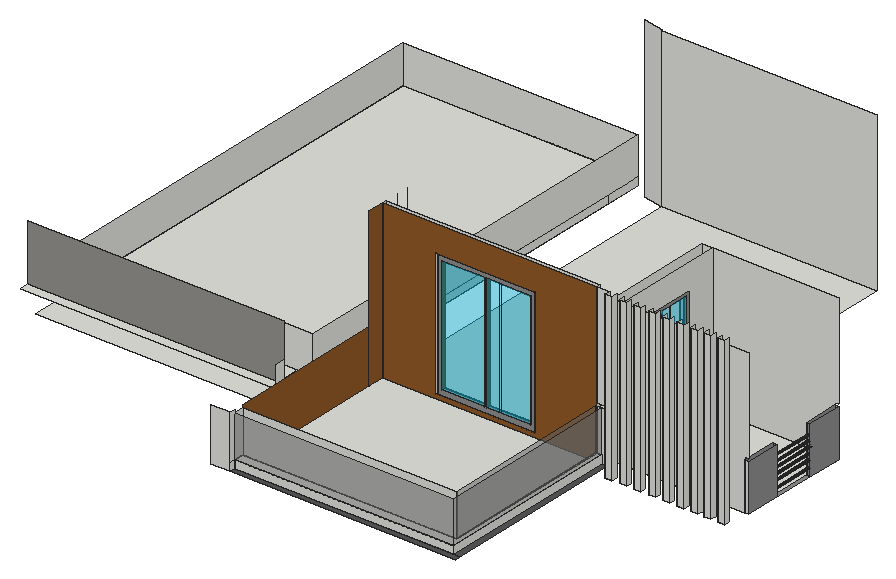
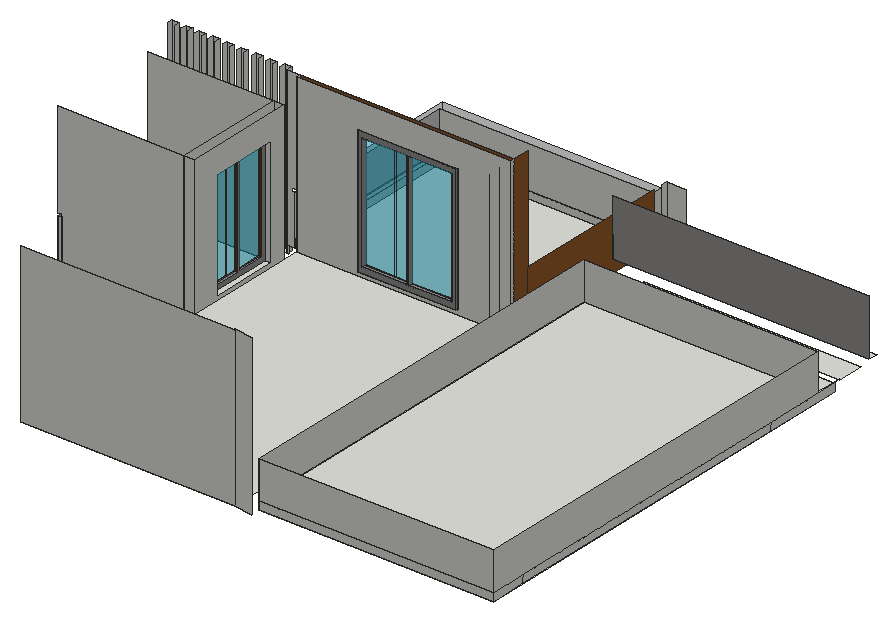
# SketchUp Ruby script. Lengths in inches.
U = 1.inch
M = Sketchup.active_model
def pt(a) = Geom::Point3d.new(a.map { |v| v * U })
def face(e, loops, mat)
  f = e.add_face(loops[0].map { |a| pt(a) })
  loops[1..].each { |l| e.add_face(l.map { |a| pt(a) }).erase! }
  f.material = f.back_material = mat if mat
  f
end
# faces: each face lists its corners as indices into pts; further lists are holes
def faces(e, pts, list, mat = nil) = list.each { |f| face(e, (f[0].is_a?(Array) ? f : [f]).map { |l| l.map { |i| pts[i] } }, mat) }
# xy, xz, yz: faces in a plane at the given z, y or x. An outline is a flat list of corners, or four numbers for a rectangle; further outlines are holes
def ring(l) = l.size == 4 ? [[l[0], l[1]], [l[2], l[1]], [l[2], l[3]], [l[0], l[3]]] : l.each_slice(2).to_a
def flat(e, list, mat, &to3) = list.each { |f| face(e, (f[0].is_a?(Array) ? f : [f]).map { |l| ring(l).map { |u, v| to3.(u, v) } }, mat) }
def xy(e, z, list, mat = nil) = flat(e, list, mat) { |x, y| [x, y, z] }
def xz(e, y, list, mat = nil) = flat(e, list, mat) { |x, z| [x, y, z] }
def yz(e, x, list, mat = nil) = flat(e, list, mat) { |y, z| [x, y, z] }
def lines(e, pts, list) = list.each { |a, b| e.add_line(pt(pts[a]), pt(pts[b])) }
# prism: a flat outline (further loops are holes) pulled along v
def prism(e, loops, v, mat = nil)
  f = face(e, loops, mat); d = Geom::Vector3d.new(v.map { |x| x * U })
  f.pushpull(f.normal.samedirection?(d) ? d.length : -d.length)
end
def box(e, o, s, mat = nil) = prism(e, [[o, [o[0] + s[0], o[1], o[2]], [o[0] + s[0], o[1] + s[1], o[2]], [o[0], o[1] + s[1], o[2]]]], [0, 0, s[2]], mat)
def at(x, y, z, deg = 0) = Geom::Transformation.translation(pt([x, y, z])) * Geom::Transformation.rotation(ORIGIN, Z_AXIS, deg.degrees)
def axes(o, x, y, z) = Geom::Transformation.new([*x, 0, *y, 0, *z, 0, *pt(o).to_a, 1])
def part(name) = M.definitions.add(name)
# library, detail: a bought-in or finely detailed component or shape, given as its bounding box
def library(name, o, s) = part(name).tap { |d| box(d.entities, o, s) }
def detail(e, o, s) = box(e.add_group.entities, o, s)
def put(e, d, t, mat = nil) = e.add_instance(d, t).tap { |i| i.material = mat if mat }
def group(e, t, mat = nil) = e.add_group.tap { |g| g.transformation = t; g.material = mat if mat }.entities
root = M.entities
M.materials.add("[Color C08]2").color = [102, 51, 0]
M.materials.add("[Color M04]").color = [142, 142, 142]
M.materials.add("[Color M06]").color = [86, 86, 86]
M.materials.add("[Color M07]").color = [58, 58, 58]
M.materials.add("[Granite Light Gray]").color = [149, 148, 144]
M.materials.add("[Translucent Glass Gray]").color = [128, 128, 128]
M.materials["[Translucent Glass Gray]"].alpha = 0.5
M.materials.add("[Translucent Glass Tinted]").color = [8, 201, 241]
M.materials["[Translucent Glass Tinted]"].alpha = 0.48
M.materials.add("[Wood Floor Parquet]").color = [145, 89, 39]
c1 = part("Group\#7")
xy(c1.entities,0,[[0,0,91.875,6]],"[Color C08]2")
xy(c1.entities,4.0625,[[4.0625,0,44.34,6],[46.04,0,87.8125,6]],"[Color M04]")
xy(c1.entities,94.75,[[4.0625,0,44.34,6],[46.04,0,87.8125,6]],"[Color M04]")
xy(c1.entities,98.8125,[[0,0,91.875,6]],"[Color M04]")
xz(c1.entities,0,[[[0,0,91.875,98.8125],[46.04,4.0625,87.8125,94.75],[4.0625,4.0625,44.34,94.75]]],"[Color M04]")
xz(c1.entities,0,[[4.0625,4.0625,44.34,94.75],[46.04,4.0625,58.41,94.75],[58.41,4.0625,60.1,94.75],[60.1,4.0625,87.8125,94.75]],"[Translucent Glass Tinted]")
xz(c1.entities,6,[[[0,0,91.875,98.8125],[46.04,4.0625,87.8125,94.75],[4.0625,4.0625,44.34,94.75]]],"[Color M04]")
yz(c1.entities,0,[[0,0,6,98.8125]],"[Color M04]")
yz(c1.entities,4.0625,[[0,4.0625,6,94.75]],"[Color C08]2")
yz(c1.entities,44.34,[[0,4.0625,6,94.75]],"[Color M04]")
yz(c1.entities,46.04,[[0,4.0625,6,94.75]],"[Color C08]2")
yz(c1.entities,87.8125,[[0,4.0625,6,94.75]],"[Color M04]")
yz(c1.entities,91.875,[[0,0,6,98.8125]],"[Color M04]")
xy(root,232.19,[[411.38,417.2,416.8,421.2],[422.38,417.2,427.8,421.2],[433.38,417.2,438.8,421.2],[444.38,417.2,449.8,421.2],[455.38,417.2,460.8,421.2],
  [466.38,417.2,471.8,421.2],[477,417.2,482.43,421.2],[487,417.2,492.43,421.2],[497.19,417.2,502.61,421.2]])
xy(root,232.48,[[503.61,435.35,506.53,462.36],[402.3125,435.41,410.3125,521],[410.3125,435.41,503.61,521],[503.61,494.13,506.53,521]])
xy(root,232.48,[[503.61,462.36,506.53,494.13]],"[Color M04]")
xy(root,234.27,[[51.29,358.3125,188.16,364.3125]])
xy(root,237.8125,[[238,280.08,238,287.59,401.5625,287.59,401.5625,421.2,405.5625,421.2,405.5625,280.08],[238,287.59,401.5625,421.2],[238,421.2,401.5625,424.01],[238,424.01,401.5625,688.37]])
xy(root,237.8125,[[238,275.76,410.3125,280.08],[405.5625,280.08,410.3125,421.2]],"[Color M06]")
xy(root,240.32,[[402.3125,448.18,410.3125,499.8]])
xy(root,241.2,[[279.03,421.2,354.66,424.01]])
xy(root,243.375,[[38.1875,364.3125,217,690.87]])
xy(root,243.8125,[[238,280.08,238,287.59,401.5625,287.59,401.5625,421.2,405.5625,421.2,405.5625,280.08],[401.36,287.59,401.5625,421.2]])
xy(root,248.4375,[[39.5625,338.43,205.18,358.3125]])
xy(root,249.375,[[38.1875,364.3125,39.5625,380.8125],[39.5625,364.3125,205.18,380.8125],[205.18,364.3125,217,380.8125],[38.1875,380.8125,217,690.87]])
xy(root,261.375,[[27.5625,338.43,223,345.62]])
xz(root,275.76,[[223,237.8125,238,278.0625]])
xz(root,280.08,[[238,237.8125,405.5625,243.8125]])
xz(root,280.08,[[238,243.8125,405.5625,276.0625]],"[Translucent Glass Gray]")
xz(root,287.59,[[238,237.8125,401.5625,243.8125],[238,243.8125,401.36,276.0625]])
xz(root,345.62,[[27.5625,261.375,223,304.375]],"[Granite Light Gray]")
xz(root,364.3125,[[38.1875,243.375,39.5625,249.375],[39.5625,243.375,205.18,249.375],[205.18,243.375,217,249.375]])
xz(root,380.8125,[[38.1875,249.375,39.5625,278.375],[39.5625,249.375,217,278.375]])
xz(root,417.2,[[411.38,232.19,416.8,357.8125],[422.38,232.19,427.8,357.8125],[433.38,232.19,438.8,357.8125],[444.38,232.19,449.8,357.8125],[455.38,232.19,460.8,357.8125],
  [466.38,232.19,471.8,357.8125],[477,232.19,482.43,357.8125],[487,232.19,492.43,357.8125],[497.19,232.19,502.61,357.8125]])
xz(root,421.2,[[410.3125,232.19,411.38,237.8125],[401.5625,237.8125,405.5625,243.8125],[405.5625,237.8125,411.38,237.8125,411.38,357.8125,401.5625,357.8125,401.5625,278.0625,407.6875,278.0625,407.6875,276.0625,405.5625,276.0625],[401.36,243.8125,401.5625,276.0625],[401.5625,243.8125,405.5625,276.0625]])
xz(root,421.2,[[[238,237.8125,401.5625,237.8125,401.5625,243.8125,401.36,243.8125,401.36,278.0625,401.5625,278.0625,401.5625,357.8125,238,357.8125],[279.03,241.2,354.66,337.83]]],"[Wood Floor Parquet]")
xz(root,424.01,[[[238,237.8125,401.5625,357.8125],[279.03,241.2,354.66,337.83]]])
xz(root,435.35,[[503.61,232.48,506.53,268.48]])
xz(root,435.41,[[402.3125,232.48,410.3125,343.15],[410.3125,232.48,410.3125,343.15,506.53,343.15,506.53,270.48,503.61,270.48,503.61,232.48]])
xz(root,448.18,[[402.3125,240.32,410.3125,323.85]])
xz(root,462.36,[[[503.61,232.48,506.53,268.48],[505.18,237.11,505.36,237.13,505.53,237.2,505.67,237.31,505.78,237.45,505.85,237.62,505.87,237.8,505.85,237.97,505.78,238.14,505.67,238.28,505.53,238.39,505.36,238.46,505.18,238.48,505.01,238.46,504.84,238.39,504.7,238.28,504.59,238.14,504.52,237.97,504.5,237.8,504.52,237.62,504.59,237.45,504.7,237.31,504.84,237.2,505.01,237.13],[505.18,264.36,505.36,264.38,505.53,264.45,505.67,264.56,505.78,264.7,505.85,264.87,505.87,265.05,505.85,265.22,505.78,265.39,505.67,265.53,505.53,265.64,505.36,265.71,505.18,265.73,505.01,265.71,504.84,265.64,504.7,265.53,504.59,265.39,504.52,265.22,504.5,265.05,504.52,264.87,504.59,264.7,504.7,264.56,504.84,264.45,505.01,264.38],[505.18,259.98,505.36,260.01,505.53,260.08,505.67,260.19,505.78,260.33,505.85,260.49,505.87,260.67,505.85,260.85,505.78,261.02,505.67,261.16,505.53,261.27,505.36,261.34,505.18,261.36,505.01,261.34,504.84,261.27,504.7,261.16,504.59,261.02,504.52,260.85,504.5,260.67,504.52,260.49,504.59,260.33,504.7,260.19,504.84,260.08,505.01,260.01],[505.18,255.61,505.36,255.63,505.53,255.7,505.67,255.81,505.78,255.95,505.85,256.12,505.87,256.3,505.85,256.47,505.78,256.64,505.67,256.78,505.53,256.89,505.36,256.96,505.18,256.98,505.01,256.96,504.84,256.89,504.7,256.78,504.59,256.64,504.52,256.47,504.5,256.3,504.52,256.12,504.59,255.95,504.7,255.81,504.84,255.7,505.01,255.63],[505.18,251.23,505.36,251.26,505.53,251.33,505.67,251.44,505.78,251.58,505.85,251.74,505.87,251.92,505.85,252.1,505.78,252.27,505.67,252.41,505.53,252.52,505.36,252.59,505.18,252.61,505.01,252.59,504.84,252.52,504.7,252.41,504.59,252.27,504.52,252.1,504.5,251.92,504.52,251.74,504.59,251.58,504.7,251.44,504.84,251.33,505.01,251.26],[505.18,246.86,505.36,246.88,505.53,246.95,505.67,247.06,505.78,247.2,505.85,247.37,505.87,247.55,505.85,247.72,505.78,247.89,505.67,248.03,505.53,248.14,505.36,248.21,505.18,248.23,505.01,248.21,504.84,248.14,504.7,248.03,504.59,247.89,504.52,247.72,504.5,247.55,504.52,247.37,504.59,247.2,504.7,247.06,504.84,246.95,505.01,246.88],[505.18,242.48,505.36,242.51,505.53,242.58,505.67,242.69,505.78,242.83,505.85,242.99,505.87,243.17,505.85,243.35,505.78,243.52,505.67,243.66,505.53,243.77,505.36,243.84,505.18,243.86,505.01,243.84,504.84,243.77,504.7,243.66,504.59,243.52,504.52,243.35,504.5,243.17,504.52,242.99,504.59,242.83,504.7,242.69,504.84,242.58,505.01,242.51]]],"[Color M04]")
xz(root,494.13,[[[503.61,232.48,506.53,268.48],[505.18,264.36,505.01,264.38,504.84,264.45,504.7,264.56,504.59,264.7,504.52,264.87,504.5,265.05,504.52,265.22,504.59,265.39,504.7,265.53,504.84,265.64,505.01,265.71,505.18,265.73,505.36,265.71,505.53,265.64,505.67,265.53,505.78,265.39,505.85,265.22,505.87,265.05,505.85,264.87,505.78,264.7,505.67,264.56,505.53,264.45,505.36,264.38],[505.18,259.98,505.01,260.01,504.84,260.08,504.7,260.19,504.59,260.33,504.52,260.49,504.5,260.67,504.52,260.85,504.59,261.02,504.7,261.16,504.84,261.27,505.01,261.34,505.18,261.36,505.36,261.34,505.53,261.27,505.67,261.16,505.78,261.02,505.85,260.85,505.87,260.67,505.85,260.49,505.78,260.33,505.67,260.19,505.53,260.08,505.36,260.01],[505.18,246.86,505.01,246.88,504.84,246.95,504.7,247.06,504.59,247.2,504.52,247.37,504.5,247.55,504.52,247.72,504.59,247.89,504.7,248.03,504.84,248.14,505.01,248.21,505.18,248.23,505.36,248.21,505.53,248.14,505.67,248.03,505.78,247.89,505.85,247.72,505.87,247.55,505.85,247.37,505.78,247.2,505.67,247.06,505.53,246.95,505.36,246.88],[505.18,242.48,505.01,242.51,504.84,242.58,504.7,242.69,504.59,242.83,504.52,242.99,504.5,243.17,504.52,243.35,504.59,243.52,504.7,243.66,504.84,243.77,505.01,243.84,505.18,243.86,505.36,243.84,505.53,243.77,505.67,243.66,505.78,243.52,505.85,243.35,505.87,243.17,505.85,242.99,505.78,242.83,505.67,242.69,505.53,242.58,505.36,242.51],[505.18,237.11,505.01,237.13,504.84,237.2,504.7,237.31,504.59,237.45,504.52,237.62,504.5,237.8,504.52,237.97,504.59,238.14,504.7,238.28,504.84,238.39,505.01,238.46,505.18,238.48,505.36,238.46,505.53,238.39,505.67,238.28,505.78,238.14,505.85,237.97,505.87,237.8,505.85,237.62,505.78,237.45,505.67,237.31,505.53,237.2,505.36,237.13]]],"[Color M04]")
xz(root,494.55,[[505.18,255.61,505.01,255.63,504.84,255.7,504.7,255.81,504.59,255.95,504.52,256.12,504.5,256.3,504.52,256.47,504.59,256.64,504.7,256.78,504.84,256.89,505.01,256.96,505.18,256.98,505.36,256.96,505.53,256.89,505.67,256.78,505.78,256.64,505.85,256.47,505.87,256.3,505.85,256.12,505.78,255.95,505.67,255.81,505.53,255.7,505.36,255.63]])
xz(root,496.55,[[505.18,251.23,505.01,251.26,504.84,251.33,504.7,251.44,504.59,251.58,504.52,251.74,504.5,251.92,504.52,252.1,504.59,252.27,504.7,252.41,504.84,252.52,505.01,252.59,505.18,252.61,505.36,252.59,505.53,252.52,505.67,252.41,505.78,252.27,505.85,252.1,505.87,251.92,505.85,251.74,505.78,251.58,505.67,251.44,505.53,251.33,505.36,251.26]])
xz(root,499.8,[[402.3125,240.32,410.3125,323.85]])
xz(root,521,[[402.3125,232.48,410.3125,343.15],[410.3125,232.48,503.61,232.48,503.61,270.48,506.53,270.48,506.53,343.15,410.3125,343.15],[503.61,232.48,506.53,268.48]])
xz(root,688.37,[[238,237.8125,401.5625,357.8125]])
xz(root,690.87,[[38.1875,243.375,217,249.375],[38.1875,249.375,217,278.375]])
yz(root,38.1875,[[364.3125,243.375,425.42,249.375],[425.42,243.375,662.42,249.375],[662.42,243.375,690.87,249.375],[380.8125,249.375,690.87,278.375]])
yz(root,217,[[364.3125,243.375,425.42,249.375],[425.42,243.375,662.42,249.375],[662.42,243.375,690.87,249.375],[380.8125,249.375,690.87,278.375]])
yz(root,223,[[338.43,261.375,345.62,278.0625]])
yz(root,238,[[275.76,237.8125,280.08,243.8125],[280.08,237.8125,287.59,243.8125],[421.2,237.8125,424.01,357.8125],[275.76,243.8125,280.08,278.0625],[280.08,243.8125,287.59,276.0625]])
yz(root,238,[[287.59,237.8125,408.45,278.0625],[408.45,237.8125,421.2,357.8125]],"[Wood Floor Parquet]")
yz(root,279.03,[[421.2,241.2,424.01,337.83]])
yz(root,354.66,[[421.2,241.2,424.01,337.83]])
yz(root,401.36,[[287.59,243.8125,421.2,276.0625]],"[Translucent Glass Gray]")
yz(root,401.5625,[[287.59,237.8125,421.2,243.8125],[421.2,237.8125,424.01,357.8125]])
yz(root,402.3125,[[[435.41,232.48,521,343.15],[448.18,240.32,499.8,323.85]]])
yz(root,405.5625,[[280.08,237.8125,421.2,243.8125]])
yz(root,405.5625,[[280.08,243.8125,421.2,276.0625]],"[Translucent Glass Gray]")
yz(root,410.3125,[[[435.41,232.48,521,343.15],[448.18,240.32,499.8,323.85]]])
yz(root,411.38,[[417.2,232.19,421.2,357.8125]])
yz(root,416.8,[[417.2,232.19,421.2,357.8125]])
yz(root,422.38,[[417.2,232.19,421.2,357.8125]])
yz(root,427.8,[[417.2,232.19,421.2,357.8125]])
yz(root,433.38,[[417.2,232.19,421.2,357.8125]])
yz(root,438.8,[[417.2,232.19,421.2,357.8125]])
yz(root,444.38,[[417.2,232.19,421.2,357.8125]])
yz(root,449.8,[[417.2,232.19,421.2,357.8125]])
yz(root,455.38,[[417.2,232.19,421.2,357.8125]])
yz(root,460.8,[[417.2,232.19,421.2,357.8125]])
yz(root,466.38,[[417.2,232.19,421.2,357.8125]])
yz(root,471.8,[[417.2,232.19,421.2,357.8125]])
yz(root,477,[[417.2,232.19,421.2,357.8125]])
yz(root,482.43,[[417.2,232.19,421.2,357.8125]])
yz(root,487,[[417.2,232.19,421.2,357.8125]])
yz(root,492.43,[[417.2,232.19,421.2,357.8125]])
yz(root,497.19,[[417.2,232.19,421.2,357.8125]])
yz(root,502.61,[[417.2,232.19,421.2,357.8125]])
yz(root,503.61,[[435.35,232.48,435.41,268.48]])
yz(root,503.61,[[435.41,232.48,462.36,268.48],[494.13,232.48,521,268.48]],"[Color M04]")
yz(root,506.53,[[435.35,232.48,462.36,268.48],[494.13,232.48,521,268.48]],"[Color M04]")
p = [[505.01,462.36,237.13],[504.84,462.36,237.2],[504.84,494.13,237.2],[505.01,494.13,237.13],[505.18,462.36,237.11],[505.18,494.13,237.11],
  [505.36,462.36,237.13],[505.36,494.13,237.13],[505.53,462.36,237.2],[505.53,494.13,237.2],[504.7,462.36,237.31],[504.7,494.13,237.31],
  [505.67,462.36,237.31],[505.67,494.13,237.31],[504.59,462.36,237.45],[504.59,494.13,237.45],[505.78,462.36,237.45],[505.78,494.13,237.45],
  [504.52,462.36,237.62],[504.52,494.13,237.62],[505.85,462.36,237.62],[505.85,494.13,237.62],[504.5,462.36,237.8],[504.5,494.13,237.8],
  [505.87,462.36,237.8],[505.87,494.13,237.8],[504.52,462.36,237.97],[504.52,494.13,237.97],[505.85,462.36,237.97],[505.85,494.13,237.97],
  [238,688.37,357.8125],[238,688.37,358.9375],[223,690.87,358.9375],[223,690.87,280.375],[223,690.87,237.8125],[238,688.37,237.8125],
  [504.59,462.36,238.14],[504.59,494.13,238.14],[505.78,462.36,238.14],[505.78,494.13,238.14],[504.7,462.36,238.28],[504.7,494.13,238.28],
  [505.67,462.36,238.28],[505.67,494.13,238.28],[504.84,462.36,238.39],[504.84,494.13,238.39],[505.53,462.36,238.39],[505.53,494.13,238.39],
  [505.01,462.36,238.46],[505.01,494.13,238.46],[505.36,462.36,238.46],[505.36,494.13,238.46],[505.18,462.36,238.48],[505.18,494.13,238.48],
  [505.01,462.36,242.51],[504.84,462.36,242.58],[504.84,494.13,242.58],[505.01,494.13,242.51],[505.18,462.36,242.48],[505.18,494.13,242.48],
  [505.36,462.36,242.51],[505.36,494.13,242.51],[505.53,462.36,242.58],[505.53,494.13,242.58],[504.7,462.36,242.69],[504.7,494.13,242.69],
  [505.67,462.36,242.69],[505.67,494.13,242.69],[504.59,462.36,242.83],[504.59,494.13,242.83],[505.78,462.36,242.83],[505.78,494.13,242.83],
  [504.52,462.36,242.99],[504.52,494.13,242.99],[505.85,462.36,242.99],[505.85,494.13,242.99],[504.5,462.36,243.17],[504.5,494.13,243.17],
  [505.87,462.36,243.17],[505.87,494.13,243.17],[504.52,462.36,243.35],[504.52,494.13,243.35],[505.85,462.36,243.35],[505.85,494.13,243.35],
  [504.59,462.36,243.52],[504.59,494.13,243.52],[505.78,462.36,243.52],[505.78,494.13,243.52],[504.7,462.36,243.66],[504.7,494.13,243.66],
  [505.67,462.36,243.66],[505.67,494.13,243.66],[504.84,462.36,243.77],[504.84,494.13,243.77],[505.53,462.36,243.77],[505.53,494.13,243.77],
  [505.01,462.36,243.84],[505.01,494.13,243.84],[505.18,462.36,243.86],[505.18,494.13,243.86],[505.36,462.36,243.84],[505.36,494.13,243.84],
  [505.01,462.36,246.88],[504.84,462.36,246.95],[504.84,494.13,246.95],[505.01,494.13,246.88],[505.18,462.36,246.86],[505.18,494.13,246.86],
  [505.36,462.36,246.88],[505.36,494.13,246.88],[505.53,462.36,246.95],[505.53,494.13,246.95],[504.7,462.36,247.06],[504.7,494.13,247.06],
  [505.67,462.36,247.06],[505.67,494.13,247.06],[504.59,462.36,247.2],[504.59,494.13,247.2],[505.78,462.36,247.2],[505.78,494.13,247.2],
  [504.52,462.36,247.37],[504.52,494.13,247.37],[505.85,462.36,247.37],[505.85,494.13,247.37],[504.5,462.36,247.55],[504.5,494.13,247.55],
  [505.87,462.36,247.55],[505.87,494.13,247.55],[504.52,462.36,247.72],[504.52,494.13,247.72],[505.85,462.36,247.72],[505.85,494.13,247.72],
  [504.59,462.36,247.89],[504.59,494.13,247.89],[505.78,462.36,247.89],[505.78,494.13,247.89],[504.7,462.36,248.03],[504.7,494.13,248.03],
  [505.67,462.36,248.03],[505.67,494.13,248.03],[504.84,462.36,248.14],[504.84,494.13,248.14],[505.53,462.36,248.14],[505.53,494.13,248.14],
  [505.01,462.36,248.21],[505.01,494.13,248.21],[505.36,462.36,248.21],[505.36,494.13,248.21],[505.18,462.36,248.23],[505.18,494.13,248.23],
  [505.18,462.36,251.23],[505.01,462.36,251.26],[505.01,496.55,251.26],[505.18,496.55,251.23],[505.36,462.36,251.26],[505.36,496.55,251.26],
  [504.84,462.36,251.33],[504.7,462.36,251.44],[504.7,496.55,251.44],[504.84,496.55,251.33],[505.53,462.36,251.33],[505.53,496.55,251.33],
  [505.67,462.36,251.44],[505.67,496.55,251.44],[504.59,462.36,251.58],[504.59,496.55,251.58],[505.78,462.36,251.58],[505.78,496.55,251.58],
  [504.52,462.36,251.74],[504.52,496.55,251.74],[505.85,462.36,251.74],[505.85,496.55,251.74],[504.5,462.36,251.92],[504.5,496.55,251.92],
  [505.87,462.36,251.92],[505.87,496.55,251.92],[504.52,462.36,252.1],[504.52,496.55,252.1],[505.85,462.36,252.1],[505.85,496.55,252.1],
  [504.59,462.36,252.27],[504.59,496.55,252.27],[505.78,462.36,252.27],[505.78,496.55,252.27],[504.7,462.36,252.41],[504.7,496.55,252.41],
  [505.67,462.36,252.41],[505.67,496.55,252.41],[504.84,462.36,252.52],[504.84,496.55,252.52],[505.53,462.36,252.52],[505.53,496.55,252.52],
  [505.01,462.36,252.59],[505.01,496.55,252.59],[505.36,462.36,252.59],[505.36,496.55,252.59],[505.18,462.36,252.61],[505.18,496.55,252.61],
  [505.01,462.36,255.63],[504.84,462.36,255.7],[504.84,494.55,255.7],[505.01,494.55,255.63],[505.18,462.36,255.61],[505.18,494.55,255.61],
  [505.36,462.36,255.63],[505.36,494.55,255.63],[505.53,462.36,255.7],[505.53,494.55,255.7],[504.7,462.36,255.81],[504.7,494.55,255.81],
  [505.67,462.36,255.81],[505.67,494.55,255.81],[504.59,462.36,255.95],[504.59,494.55,255.95],[505.78,462.36,255.95],[505.78,494.55,255.95],
  [504.52,462.36,256.12],[504.52,494.55,256.12],[505.85,462.36,256.12],[505.85,494.55,256.12],[504.5,462.36,256.3],[504.5,494.55,256.3],
  [505.87,462.36,256.3],[505.87,494.55,256.3],[504.52,462.36,256.47],[504.52,494.55,256.47],[505.85,462.36,256.47],[505.85,494.55,256.47],
  [504.59,462.36,256.64],[504.59,494.55,256.64],[505.78,462.36,256.64],[505.78,494.55,256.64],[504.7,462.36,256.78],[504.7,494.55,256.78],
  [505.67,462.36,256.78],[505.67,494.55,256.78],[504.84,462.36,256.89],[504.84,494.55,256.89],[505.53,462.36,256.89],[505.53,494.55,256.89],
  [505.01,462.36,256.96],[505.01,494.55,256.96],[505.36,462.36,256.96],[505.36,494.55,256.96],[505.18,462.36,256.98],[505.18,494.55,256.98],
  [505.01,462.36,260.01],[504.84,462.36,260.08],[504.84,494.13,260.08],[505.01,494.13,260.01],[505.18,462.36,259.98],[505.18,494.13,259.98],
  [505.36,462.36,260.01],[505.36,494.13,260.01],[505.53,462.36,260.08],[505.53,494.13,260.08],[504.7,462.36,260.19],[504.7,494.13,260.19],
  [505.67,462.36,260.19],[505.67,494.13,260.19],[504.59,462.36,260.33],[504.59,494.13,260.33],[505.78,462.36,260.33],[505.78,494.13,260.33],
  [504.52,462.36,260.49],[504.52,494.13,260.49],[505.85,462.36,260.49],[505.85,494.13,260.49],[504.5,462.36,260.67],[504.5,494.13,260.67],
  [505.87,462.36,260.67],[505.87,494.13,260.67],[504.52,462.36,260.85],[504.52,494.13,260.85],[505.85,462.36,260.85],[505.85,494.13,260.85],
  [504.59,462.36,261.02],[504.59,494.13,261.02],[505.78,462.36,261.02],[505.78,494.13,261.02],[504.7,462.36,261.16],[504.7,494.13,261.16],
  [505.67,462.36,261.16],[505.67,494.13,261.16],[504.84,462.36,261.27],[504.84,494.13,261.27],[505.53,462.36,261.27],[505.53,494.13,261.27],
  [505.01,462.36,261.34],[505.01,494.13,261.34],[505.18,462.36,261.36],[505.18,494.13,261.36],[505.36,462.36,261.34],[505.36,494.13,261.34],
  [205.18,358.3125,249.375],[205.18,364.3125,249.375],[39.5625,358.3125,249.375],[39.5625,364.3125,249.375],[238,408.45,237.8125],[238.25,408.45,237.8125],
  [238,435,237.8125],[238,435,357.8125],[238,445.125,237.8125],[238,445.125,357.8125]]
faces(root,p,[[0,1,2,3],[4,0,3,5],[6,4,5,7],[8,6,7,9],[1,10,11,2],[12,8,9,13],[10,14,15,11],[16,12,13,17],
  [14,18,19,15],[20,16,17,21],[18,22,23,19],[24,20,21,25],[22,26,27,23],[28,24,25,29],[26,36,37,27],[38,28,29,39],
  [36,40,41,37],[42,38,39,43],[40,44,45,41],[46,42,43,47],[44,48,49,45],[50,46,47,51],[48,52,53,49],[52,50,51,53],
  [54,55,56,57],[58,54,57,59],[60,58,59,61],[62,60,61,63],[55,64,65,56],[66,62,63,67],[64,68,69,65],[70,66,67,71],
  [68,72,73,69],[74,70,71,75],[72,76,77,73],[78,74,75,79],[76,80,81,77],[82,78,79,83],[80,84,85,81],[86,82,83,87],
  [84,88,89,85],[90,86,87,91],[88,92,93,89],[94,90,91,95],[92,96,97,93],[96,98,99,97],[98,100,101,99],[100,94,95,101],
  [102,103,104,105],[106,102,105,107],[108,106,107,109],[110,108,109,111],[103,112,113,104],[114,110,111,115],[112,116,117,113],[118,114,115,119],
  [116,120,121,117],[122,118,119,123],[120,124,125,121],[126,122,123,127],[124,128,129,125],[130,126,127,131],[128,132,133,129],[134,130,131,135],
  [132,136,137,133],[138,134,135,139],[136,140,141,137],[142,138,139,143],[140,144,145,141],[146,142,143,147],[144,148,149,145],[148,146,147,149],
  [150,151,152,153],[154,150,153,155],[156,157,158,159],[151,156,159,152],[160,154,155,161],[162,160,161,163],[157,164,165,158],[166,162,163,167],
  [164,168,169,165],[170,166,167,171],[168,172,173,169],[174,170,171,175],[172,176,177,173],[178,174,175,179],[176,180,181,177],[182,178,179,183],
  [180,184,185,181],[186,182,183,187],[184,188,189,185],[190,186,187,191],[188,192,193,189],[194,190,191,195],[192,196,197,193],[196,194,195,197],
  [198,199,200,201],[202,198,201,203],[204,202,203,205],[206,204,205,207],[199,208,209,200],[210,206,207,211],[208,212,213,209],[214,210,211,215],
  [212,216,217,213],[218,214,215,219],[216,220,221,217],[222,218,219,223],[220,224,225,221],[226,222,223,227],[224,228,229,225],[230,226,227,231],
  [228,232,233,229],[234,230,231,235],[232,236,237,233],[238,234,235,239],[236,240,241,237],[242,238,239,243],[240,244,245,241],[244,242,243,245],
  [246,247,248,249],[250,246,249,251],[252,250,251,253],[254,252,253,255],[247,256,257,248],[258,254,255,259],[256,260,261,257],[262,258,259,263],
  [260,264,265,261],[266,262,263,267],[264,268,269,265],[270,266,267,271],[268,272,273,269],[274,270,271,275],[272,276,277,273],[278,274,275,279],
  [276,280,281,277],[282,278,279,283],[280,284,285,281],[286,282,283,287],[284,288,289,285],[288,290,291,289],[290,292,293,291],[292,286,287,293]],"[Color M07]")
faces(root,p,[[30,31,32,33,34,35]])
lines(root,p,[[294,295],[296,297],[298,299],[300,301],[302,303]])
put(root,c1,axes([409.53,448.18,240.32],[0,0.5619,0],[-0.41307,0,0],[0,0,0.84535]))
put(root,c1,axes([279.76,421.41,241.2],[0.81526,0,0],[0,0.54351,0],[0,0,0.97786]))
